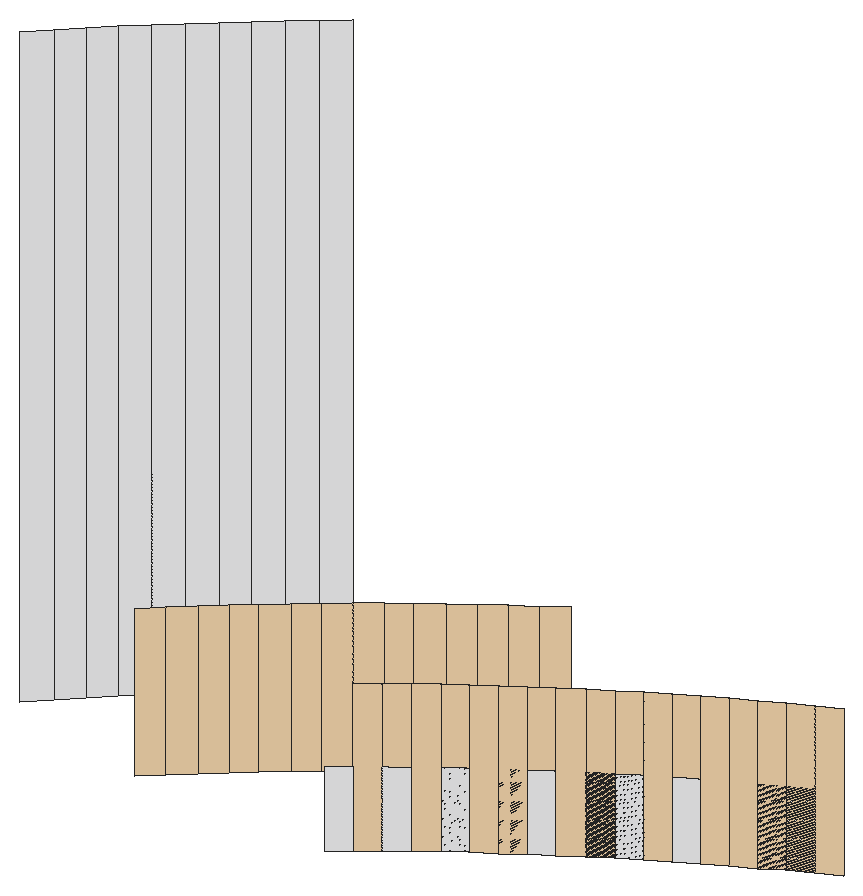
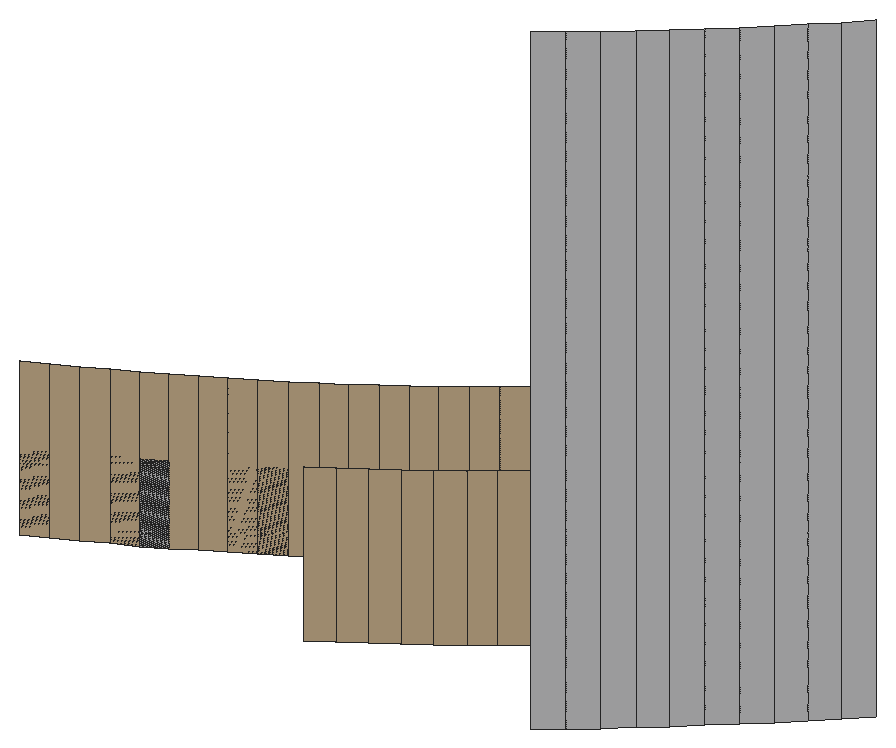
# SketchUp Ruby script. Lengths in inches.
U = 1.inch
M = Sketchup.active_model
def pt(a) = Geom::Point3d.new(a.map { |v| v * U })
def face(e, loops, mat)
  f = e.add_face(loops[0].map { |a| pt(a) })
  loops[1..].each { |l| e.add_face(l.map { |a| pt(a) }).erase! }
  f.material = f.back_material = mat if mat
  f
end
# faces: each face lists its corners as indices into pts; further lists are holes
def faces(e, pts, list, mat = nil) = list.each { |f| face(e, (f[0].is_a?(Array) ? f : [f]).map { |l| l.map { |i| pts[i] } }, mat) }
# xy, xz, yz: faces in a plane at the given z, y or x. An outline is a flat list of corners, or four numbers for a rectangle; further outlines are holes
def ring(l) = l.size == 4 ? [[l[0], l[1]], [l[2], l[1]], [l[2], l[3]], [l[0], l[3]]] : l.each_slice(2).to_a
def flat(e, list, mat, &to3) = list.each { |f| face(e, (f[0].is_a?(Array) ? f : [f]).map { |l| ring(l).map { |u, v| to3.(u, v) } }, mat) }
def xy(e, z, list, mat = nil) = flat(e, list, mat) { |x, y| [x, y, z] }
def xz(e, y, list, mat = nil) = flat(e, list, mat) { |x, z| [x, y, z] }
def yz(e, x, list, mat = nil) = flat(e, list, mat) { |y, z| [x, y, z] }
def lines(e, pts, list) = list.each { |a, b| e.add_line(pt(pts[a]), pt(pts[b])) }
# prism: a flat outline (further loops are holes) pulled along v
def prism(e, loops, v, mat = nil)
  f = face(e, loops, mat); d = Geom::Vector3d.new(v.map { |x| x * U })
  f.pushpull(f.normal.samedirection?(d) ? d.length : -d.length)
end
def box(e, o, s, mat = nil) = prism(e, [[o, [o[0] + s[0], o[1], o[2]], [o[0] + s[0], o[1] + s[1], o[2]], [o[0], o[1] + s[1], o[2]]]], [0, 0, s[2]], mat)
def at(x, y, z, deg = 0) = Geom::Transformation.translation(pt([x, y, z])) * Geom::Transformation.rotation(ORIGIN, Z_AXIS, deg.degrees)
def axes(o, x, y, z) = Geom::Transformation.new([*x, 0, *y, 0, *z, 0, *pt(o).to_a, 1])
def part(name) = M.definitions.add(name)
# library, detail: a bought-in or finely detailed component or shape, given as its bounding box
def library(name, o, s) = part(name).tap { |d| box(d.entities, o, s) }
def detail(e, o, s) = box(e.add_group.entities, o, s)
def put(e, d, t, mat = nil) = e.add_instance(d, t).tap { |i| i.material = mat if mat }
def group(e, t, mat = nil) = e.add_group.tap { |g| g.transformation = t; g.material = mat if mat }.entities
root = M.entities
M.materials.add("False Ceiling Light").color = [254, 223, 179]
M.materials.add("[Quartz Light Grey]").color = [251, 251, 252]
p = [[47.02,214.52,115.32],[46.88,214.39,115.32],[46.88,214.39,116.49],[47.02,214.52,116.49],[48.5,214.49,115.32],[48.37,214.38,115.32],
  [48.37,214.38,115.91],[48.5,214.49,115.91],[47.16,214.65,115.32],[47.16,214.65,116.49],[48.64,214.6,115.32],[48.64,214.6,115.91],
  [48.5,214.49,115.32],[48.64,214.6,115.32],[48.64,214.6,116.49],[48.5,214.49,116.49],[47.3,214.78,115.32],[47.3,214.78,116.49],
  [48.78,214.71,115.32],[48.78,214.71,115.91],[48.78,214.71,115.32],[48.78,214.71,116.49],[45.76,214.67,115.32],[45.9,214.82,115.32],
  [45.9,214.82,120],[45.76,214.67,120],[48.92,214.82,115.32],[48.92,214.82,115.91],[48.92,214.82,115.32],[48.92,214.82,116.49],
  [46.04,214.96,115.32],[46.04,214.96,120],[47.4375,214.9,115.32],[47.4375,214.9,116.49],[49.06,214.92,115.32],[49.06,214.92,115.91],
  [49.06,214.92,115.32],[49.06,214.92,116.49],[47.58,215.03,115.32],[47.58,215.03,116.49],[49.21,215.02,115.32],[49.21,215.02,115.91],
  [49.21,215.02,115.32],[49.21,215.02,116.49],[46.18,215.1,115.32],[46.18,215.1,120],[47.73,215.15,115.32],[47.73,215.15,116.49],
  [49.35,215.125,115.32],[49.35,215.125,115.91],[49.35,215.125,115.32],[49.35,215.125,116.49],[46.33,215.24,115.32],[46.33,215.24,120],
  [47.875,215.27,115.32],[47.875,215.27,116.49],[49.5,215.22,115.32],[49.5,215.22,115.91],[49.5,215.22,115.32],[49.5,215.22,116.49],
  [46.48,215.38,115.32],[46.48,215.38,120],[49.65,215.32,115.32],[49.65,215.32,115.91],[49.65,215.32,115.32],[49.65,215.32,116.49],
  [48.02,215.39,115.32],[48.02,215.39,116.49],[49.8,215.42,115.32],[49.8,215.42,115.91],[49.8,215.42,115.32],[49.8,215.42,116.49],
  [46.63,215.52,115.32],[46.63,215.52,120],[48.17,215.5,115.32],[48.17,215.5,116.49],[49.95,215.51,115.32],[49.95,215.51,115.91],
  [49.95,215.51,115.32],[49.95,215.51,116.49],[46.78,215.65,115.32],[46.78,215.65,120],[48.32,215.62,115.32],[48.32,215.62,116.49],
  [50.1,215.6,115.32],[50.1,215.6,115.91],[50.1,215.6,115.32],[50.1,215.6,116.49],[48.48,215.73,115.32],[48.48,215.73,116.49],
  [50.25,215.69,115.32],[50.25,215.69,115.91],[50.25,215.69,115.32],[50.25,215.69,116.49],[46.93,215.79,115.32],[46.93,215.79,120],
  [48.63,215.84,115.32],[48.63,215.84,116.49],[50.4,215.78,115.32],[50.4,215.78,115.91],[50.4,215.78,115.32],[50.4,215.78,116.49],
  [47.09,215.92,115.32],[47.09,215.92,120],[48.79,215.95,115.32],[48.79,215.95,116.49],[50.56,215.86,115.32],[50.56,215.86,115.91],
  [50.56,215.86,115.32],[50.56,215.86,116.49],[47.25,216.05,115.32],[47.25,216.05,120],[48.94,216.06,115.32],[48.94,216.06,116.49],
  [50.71,215.95,115.32],[50.71,215.95,115.91],[50.71,215.95,115.32],[50.71,215.95,116.49],[50.87,216.03,115.32],[50.87,216.03,115.91],
  [50.87,216.03,115.32],[50.87,216.03,116.49],[51.03,216.11,115.32],[51.03,216.11,115.91],[51.03,216.11,115.32],[51.03,216.11,116.49]]
faces(root,p,[[0,1,2,3],[8,0,3,9],[12,13,14,15],[16,8,9,17],[13,20,21,14],[20,28,29,21],[32,16,17,33],[28,36,37,29],
  [38,32,33,39],[36,42,43,37],[46,38,39,47],[42,50,51,43],[54,46,47,55],[50,58,59,51],[58,64,65,59],[66,54,55,67],
  [64,70,71,65],[74,66,67,75],[70,78,79,71],[82,74,75,83],[78,86,87,79],[88,82,83,89],[86,92,93,87],[96,88,89,97],
  [92,100,101,93],[104,96,97,105],[100,108,109,101],[112,104,105,113],[108,116,117,109],[116,120,121,117],[120,124,125,121]],"False Ceiling Light")
faces(root,p,[[4,5,6,7],[10,4,7,11],[18,10,11,19],[22,23,24,25],[26,18,19,27],[23,30,31,24],[34,26,27,35],[40,34,35,41],
  [30,44,45,31],[48,40,41,49],[44,52,53,45],[56,48,49,57],[52,60,61,53],[62,56,57,63],[68,62,63,69],[60,72,73,61],
  [76,68,69,77],[72,80,81,73],[84,76,77,85],[90,84,85,91],[80,94,95,81],[98,90,91,99],[94,102,103,95],[106,98,99,107],
  [102,110,111,103],[114,106,107,115],[118,114,115,119],[122,118,119,123]],"[Quartz Light Grey]")
